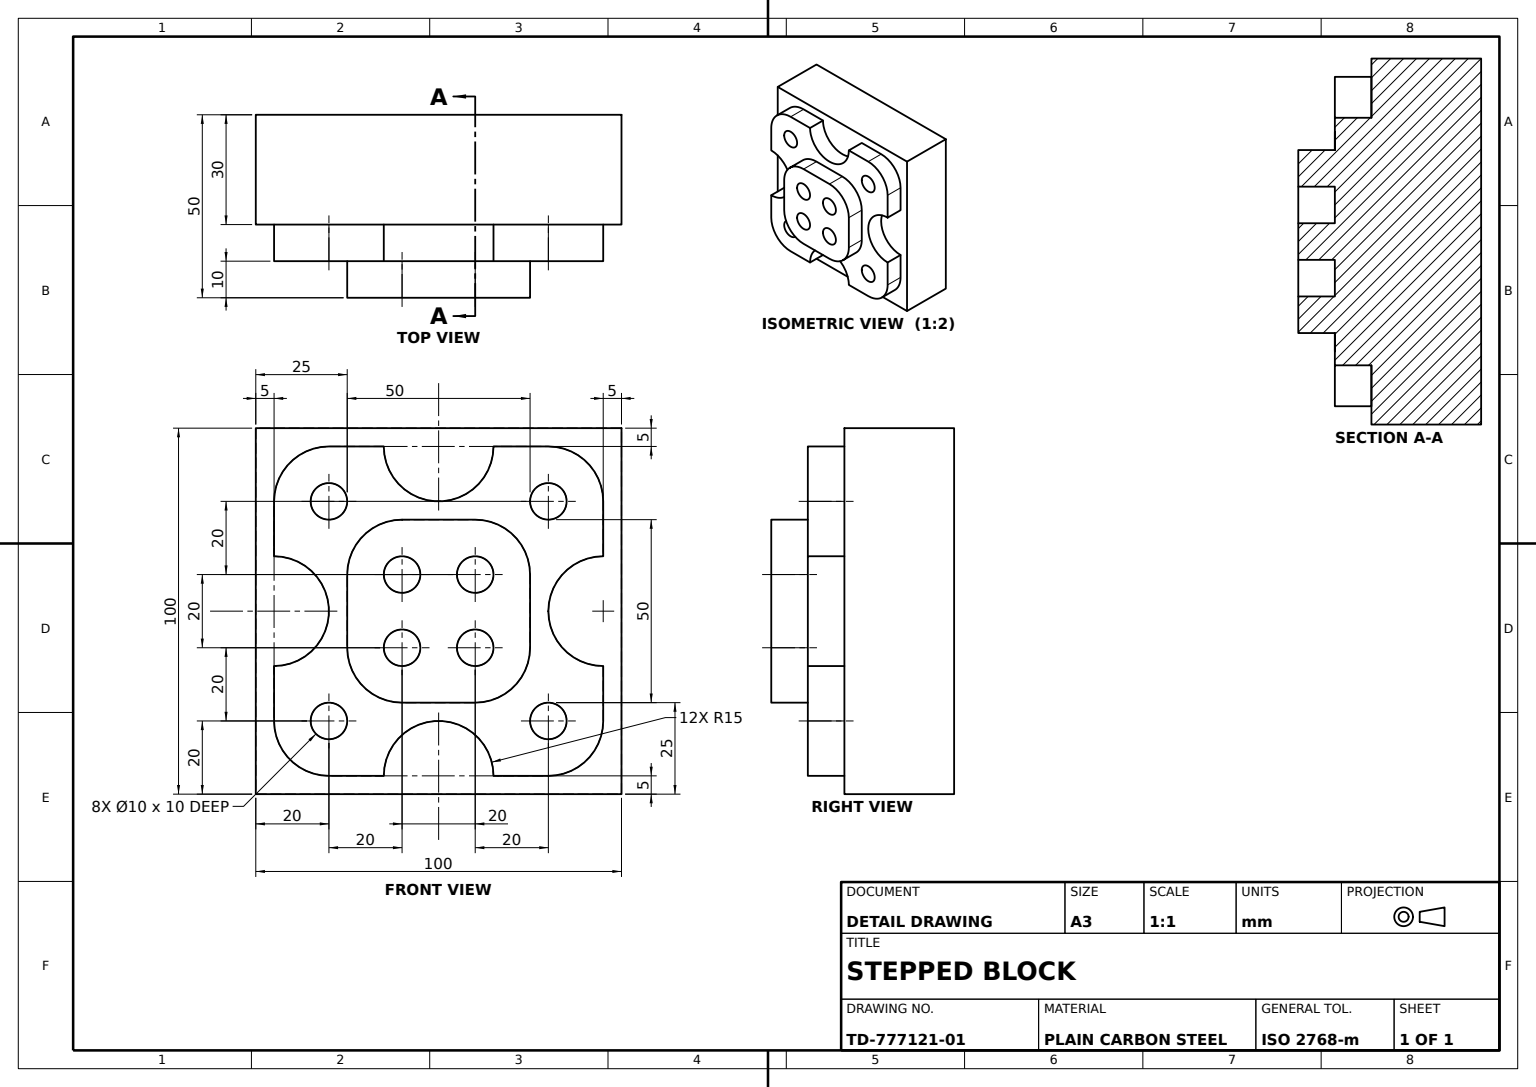
ISO-10303-21;
HEADER;
FILE_DESCRIPTION((''),'2;1');
FILE_NAME('','',(''),(''),'','','');
FILE_SCHEMA(('AUTOMOTIVE_DESIGN'));
ENDSEC;
DATA;
#1=APPLICATION_CONTEXT('');
#2=PRODUCT_CONTEXT('',#1,'mechanical');
#3=PRODUCT('','','',(#2));
#4=PRODUCT_DEFINITION_FORMATION('','',#3);
#5=PRODUCT_DEFINITION_CONTEXT('',#1,'design');
#6=PRODUCT_DEFINITION('','',#4,#5);
#7=PRODUCT_DEFINITION_SHAPE('','',#6);
#8=(LENGTH_UNIT()NAMED_UNIT(*)SI_UNIT(.MILLI.,.METRE.));
#9=(NAMED_UNIT(*)PLANE_ANGLE_UNIT()SI_UNIT($,.RADIAN.));
#10=(NAMED_UNIT(*)SI_UNIT($,.STERADIAN.)SOLID_ANGLE_UNIT());
#11=UNCERTAINTY_MEASURE_WITH_UNIT(LENGTH_MEASURE(1.E-05),#8,'distance_accuracy_value','');
#12=(GEOMETRIC_REPRESENTATION_CONTEXT(3)GLOBAL_UNCERTAINTY_ASSIGNED_CONTEXT((#11))GLOBAL_UNIT_ASSIGNED_CONTEXT((#8,#9,#10))REPRESENTATION_CONTEXT('',''));
#13=CARTESIAN_POINT('',(35.,-5.,30.));
#14=VERTEX_POINT('',#13);
#15=CARTESIAN_POINT('',(20.,-5.,30.));
#16=VERTEX_POINT('',#15);
#17=DIRECTION('',(-1.,0.,0.));
#18=VECTOR('',#17,1000.);
#19=LINE('',#15,#18);
#20=EDGE_CURVE('',#14,#16,#19,.T.);
#21=ORIENTED_EDGE('',*,*,#20,.T.);
#22=CARTESIAN_POINT('',(20.,-5.,40.));
#23=VERTEX_POINT('',#22);
#24=DIRECTION('',(0.,0.,-1.));
#25=VECTOR('',#24,1000.);
#26=LINE('',#22,#25);
#27=EDGE_CURVE('',#23,#16,#26,.T.);
#28=ORIENTED_EDGE('',*,*,#27,.F.);
#29=CARTESIAN_POINT('',(35.,-5.,40.));
#30=VERTEX_POINT('',#29);
#31=LINE('',#22,#18);
#32=EDGE_CURVE('',#30,#23,#31,.T.);
#33=ORIENTED_EDGE('',*,*,#32,.F.);
#34=LINE('',#29,#25);
#35=EDGE_CURVE('',#30,#14,#34,.T.);
#36=ORIENTED_EDGE('',*,*,#35,.T.);
#37=EDGE_LOOP('',(#21,#28,#33,#36));
#38=FACE_OUTER_BOUND('',#37,.T.);
#39=DIRECTION('',(0.,-1.,0.));
#40=AXIS2_PLACEMENT_3D('',#22,#39,#24);
#41=PLANE('',#40);
#42=ADVANCED_FACE('',(#38),#41,.F.);
#43=CARTESIAN_POINT('',(25.,-40.,40.));
#44=VERTEX_POINT('',#43);
#45=CARTESIAN_POINT('',(25.,-60.,40.));
#46=VERTEX_POINT('',#45);
#47=VECTOR('',#39,1000.);
#48=LINE('',#43,#47);
#49=EDGE_CURVE('',#44,#46,#48,.T.);
#50=ORIENTED_EDGE('',*,*,#49,.T.);
#51=CARTESIAN_POINT('',(25.,-60.,50.));
#52=VERTEX_POINT('',#51);
#53=LINE('',#51,#25);
#54=EDGE_CURVE('',#52,#46,#53,.T.);
#55=ORIENTED_EDGE('',*,*,#54,.F.);
#56=CARTESIAN_POINT('',(25.,-40.,50.));
#57=VERTEX_POINT('',#56);
#58=LINE('',#56,#47);
#59=EDGE_CURVE('',#57,#52,#58,.T.);
#60=ORIENTED_EDGE('',*,*,#59,.F.);
#61=LINE('',#56,#25);
#62=EDGE_CURVE('',#57,#44,#61,.T.);
#63=ORIENTED_EDGE('',*,*,#62,.T.);
#64=EDGE_LOOP('',(#50,#55,#60,#63));
#65=FACE_OUTER_BOUND('',#64,.T.);
#66=DIRECTION('',(1.,0.,0.));
#67=DIRECTION('',(0.,1.,0.));
#68=AXIS2_PLACEMENT_3D('',#56,#66,#67);
#69=PLANE('',#68);
#70=ADVANCED_FACE('',(#65),#69,.F.);
#71=CARTESIAN_POINT('',(75.,-20.,30.));
#72=VERTEX_POINT('',#71);
#73=CARTESIAN_POINT('',(75.,-20.,40.));
#74=VERTEX_POINT('',#73);
#75=DIRECTION('',(0.,0.,1.));
#76=VECTOR('',#75,1000.);
#77=LINE('',#71,#76);
#78=EDGE_CURVE('',#72,#74,#77,.T.);
#79=ORIENTED_EDGE('',*,*,#78,.T.);
#80=CARTESIAN_POINT('',(85.,-20.,40.));
#81=VERTEX_POINT('',#80);
#82=CARTESIAN_POINT('',(80.,-20.,40.));
#83=AXIS2_PLACEMENT_3D('',#82,#75,#66);
#84=CIRCLE('',#83,5.);
#85=EDGE_CURVE('',#74,#81,#84,.T.);
#86=ORIENTED_EDGE('',*,*,#85,.T.);
#87=CARTESIAN_POINT('',(85.,-20.,30.));
#88=VERTEX_POINT('',#87);
#89=LINE('',#87,#76);
#90=EDGE_CURVE('',#88,#81,#89,.T.);
#91=ORIENTED_EDGE('',*,*,#90,.F.);
#92=CARTESIAN_POINT('',(80.,-20.,30.));
#93=AXIS2_PLACEMENT_3D('',#92,#75,#66);
#94=CIRCLE('',#93,5.);
#95=EDGE_CURVE('',#72,#88,#94,.T.);
#96=ORIENTED_EDGE('',*,*,#95,.F.);
#97=EDGE_LOOP('',(#79,#86,#91,#96));
#98=FACE_OUTER_BOUND('',#97,.T.);
#99=CYLINDRICAL_SURFACE('',#93,5.);
#100=ADVANCED_FACE('',(#98),#99,.F.);
#101=CARTESIAN_POINT('',(65.,-5.,40.));
#102=VERTEX_POINT('',#101);
#103=CARTESIAN_POINT('',(50.,-5.,40.));
#104=AXIS2_PLACEMENT_3D('',#103,#24,#66);
#105=CIRCLE('',#104,15.);
#106=EDGE_CURVE('',#102,#30,#105,.T.);
#107=ORIENTED_EDGE('',*,*,#106,.F.);
#108=CARTESIAN_POINT('',(65.,-5.,30.));
#109=VERTEX_POINT('',#108);
#110=LINE('',#101,#25);
#111=EDGE_CURVE('',#102,#109,#110,.T.);
#112=ORIENTED_EDGE('',*,*,#111,.T.);
#113=CARTESIAN_POINT('',(50.,-5.,30.));
#114=AXIS2_PLACEMENT_3D('',#113,#24,#66);
#115=CIRCLE('',#114,15.);
#116=EDGE_CURVE('',#109,#14,#115,.T.);
#117=ORIENTED_EDGE('',*,*,#116,.T.);
#118=ORIENTED_EDGE('',*,*,#35,.F.);
#119=EDGE_LOOP('',(#107,#112,#117,#118));
#120=FACE_OUTER_BOUND('',#119,.T.);
#121=AXIS2_PLACEMENT_3D('',#103,#24,#17);
#122=CYLINDRICAL_SURFACE('',#121,15.);
#123=ADVANCED_FACE('',(#120),#122,.F.);
#124=CARTESIAN_POINT('',(65.,-40.,40.));
#125=VERTEX_POINT('',#124);
#126=CARTESIAN_POINT('',(55.,-40.,40.));
#127=VERTEX_POINT('',#126);
#128=CARTESIAN_POINT('',(60.,-40.,40.));
#129=AXIS2_PLACEMENT_3D('',#128,#75,#66);
#130=CIRCLE('',#129,5.);
#131=EDGE_CURVE('',#125,#127,#130,.T.);
#132=ORIENTED_EDGE('',*,*,#131,.T.);
#133=EDGE_CURVE('',#127,#125,#130,.T.);
#134=ORIENTED_EDGE('',*,*,#133,.T.);
#135=EDGE_LOOP('',(#132,#134));
#136=FACE_OUTER_BOUND('',#135,.T.);
#137=PLANE('',#129);
#138=ADVANCED_FACE('',(#136),#137,.T.);
#139=CARTESIAN_POINT('',(80.,-5.,30.));
#140=VERTEX_POINT('',#139);
#141=LINE('',#108,#18);
#142=EDGE_CURVE('',#140,#109,#141,.T.);
#143=ORIENTED_EDGE('',*,*,#142,.T.);
#144=ORIENTED_EDGE('',*,*,#111,.F.);
#145=CARTESIAN_POINT('',(80.,-5.,40.));
#146=VERTEX_POINT('',#145);
#147=LINE('',#101,#18);
#148=EDGE_CURVE('',#146,#102,#147,.T.);
#149=ORIENTED_EDGE('',*,*,#148,.F.);
#150=LINE('',#145,#25);
#151=EDGE_CURVE('',#146,#140,#150,.T.);
#152=ORIENTED_EDGE('',*,*,#151,.T.);
#153=EDGE_LOOP('',(#143,#144,#149,#152));
#154=FACE_OUTER_BOUND('',#153,.T.);
#155=AXIS2_PLACEMENT_3D('',#101,#39,#24);
#156=PLANE('',#155);
#157=ADVANCED_FACE('',(#154),#156,.F.);
#158=CARTESIAN_POINT('',(85.,-80.,40.));
#159=VERTEX_POINT('',#158);
#160=CARTESIAN_POINT('',(75.,-80.,40.));
#161=VERTEX_POINT('',#160);
#162=CARTESIAN_POINT('',(80.,-80.,40.));
#163=AXIS2_PLACEMENT_3D('',#162,#75,#66);
#164=CIRCLE('',#163,5.);
#165=EDGE_CURVE('',#159,#161,#164,.T.);
#166=ORIENTED_EDGE('',*,*,#165,.T.);
#167=CARTESIAN_POINT('',(75.,-80.,30.));
#168=VERTEX_POINT('',#167);
#169=LINE('',#167,#76);
#170=EDGE_CURVE('',#168,#161,#169,.T.);
#171=ORIENTED_EDGE('',*,*,#170,.F.);
#172=CARTESIAN_POINT('',(85.,-80.,30.));
#173=VERTEX_POINT('',#172);
#174=CARTESIAN_POINT('',(80.,-80.,30.));
#175=AXIS2_PLACEMENT_3D('',#174,#75,#66);
#176=CIRCLE('',#175,5.);
#177=EDGE_CURVE('',#173,#168,#176,.T.);
#178=ORIENTED_EDGE('',*,*,#177,.F.);
#179=LINE('',#172,#76);
#180=EDGE_CURVE('',#173,#159,#179,.T.);
#181=ORIENTED_EDGE('',*,*,#180,.T.);
#182=EDGE_LOOP('',(#166,#171,#178,#181));
#183=FACE_OUTER_BOUND('',#182,.T.);
#184=CYLINDRICAL_SURFACE('',#175,5.);
#185=ADVANCED_FACE('',(#183),#184,.F.);
#186=CARTESIAN_POINT('',(40.,-75.,50.));
#187=VERTEX_POINT('',#186);
#188=CARTESIAN_POINT('',(60.,-75.,50.));
#189=VERTEX_POINT('',#188);
#190=VECTOR('',#66,1000.);
#191=LINE('',#186,#190);
#192=EDGE_CURVE('',#187,#189,#191,.T.);
#193=ORIENTED_EDGE('',*,*,#192,.F.);
#194=CARTESIAN_POINT('',(40.,-75.,40.));
#195=VERTEX_POINT('',#194);
#196=LINE('',#186,#25);
#197=EDGE_CURVE('',#187,#195,#196,.T.);
#198=ORIENTED_EDGE('',*,*,#197,.T.);
#199=CARTESIAN_POINT('',(60.,-75.,40.));
#200=VERTEX_POINT('',#199);
#201=LINE('',#194,#190);
#202=EDGE_CURVE('',#195,#200,#201,.T.);
#203=ORIENTED_EDGE('',*,*,#202,.T.);
#204=LINE('',#188,#25);
#205=EDGE_CURVE('',#189,#200,#204,.T.);
#206=ORIENTED_EDGE('',*,*,#205,.F.);
#207=EDGE_LOOP('',(#193,#198,#203,#206));
#208=FACE_OUTER_BOUND('',#207,.T.);
#209=AXIS2_PLACEMENT_3D('',#186,#67,#75);
#210=PLANE('',#209);
#211=ADVANCED_FACE('',(#208),#210,.F.);
#212=CARTESIAN_POINT('',(100.,-100.,30.));
#213=VERTEX_POINT('',#212);
#214=CARTESIAN_POINT('',(100.,0.,30.));
#215=VERTEX_POINT('',#214);
#216=VECTOR('',#67,1000.);
#217=LINE('',#212,#216);
#218=EDGE_CURVE('',#213,#215,#217,.T.);
#219=ORIENTED_EDGE('',*,*,#218,.T.);
#220=CARTESIAN_POINT('',(0.,0.,30.));
#221=VERTEX_POINT('',#220);
#222=LINE('',#214,#18);
#223=EDGE_CURVE('',#215,#221,#222,.T.);
#224=ORIENTED_EDGE('',*,*,#223,.T.);
#225=CARTESIAN_POINT('',(0.,-100.,30.));
#226=VERTEX_POINT('',#225);
#227=LINE('',#220,#47);
#228=EDGE_CURVE('',#221,#226,#227,.T.);
#229=ORIENTED_EDGE('',*,*,#228,.T.);
#230=LINE('',#225,#190);
#231=EDGE_CURVE('',#226,#213,#230,.T.);
#232=ORIENTED_EDGE('',*,*,#231,.T.);
#233=EDGE_LOOP('',(#219,#224,#229,#232));
#234=FACE_OUTER_BOUND('',#233,.T.);
#235=CARTESIAN_POINT('',(5.,-20.,30.));
#236=VERTEX_POINT('',#235);
#237=CARTESIAN_POINT('',(5.,-35.,30.));
#238=VERTEX_POINT('',#237);
#239=LINE('',#235,#47);
#240=EDGE_CURVE('',#236,#238,#239,.T.);
#241=ORIENTED_EDGE('',*,*,#240,.F.);
#242=CARTESIAN_POINT('',(20.,-20.,30.));
#243=AXIS2_PLACEMENT_3D('',#242,#75,#66);
#244=CIRCLE('',#243,15.);
#245=EDGE_CURVE('',#16,#236,#244,.T.);
#246=ORIENTED_EDGE('',*,*,#245,.F.);
#247=ORIENTED_EDGE('',*,*,#20,.F.);
#248=ORIENTED_EDGE('',*,*,#116,.F.);
#249=ORIENTED_EDGE('',*,*,#142,.F.);
#250=CARTESIAN_POINT('',(95.,-20.,30.));
#251=VERTEX_POINT('',#250);
#252=CIRCLE('',#93,15.);
#253=EDGE_CURVE('',#251,#140,#252,.T.);
#254=ORIENTED_EDGE('',*,*,#253,.F.);
#255=CARTESIAN_POINT('',(95.,-35.,30.));
#256=VERTEX_POINT('',#255);
#257=LINE('',#250,#216);
#258=EDGE_CURVE('',#256,#251,#257,.T.);
#259=ORIENTED_EDGE('',*,*,#258,.F.);
#260=CARTESIAN_POINT('',(80.,-50.,30.));
#261=VERTEX_POINT('',#260);
#262=CARTESIAN_POINT('',(95.,-50.,30.));
#263=AXIS2_PLACEMENT_3D('',#262,#24,#66);
#264=CIRCLE('',#263,15.);
#265=EDGE_CURVE('',#261,#256,#264,.T.);
#266=ORIENTED_EDGE('',*,*,#265,.F.);
#267=CARTESIAN_POINT('',(95.,-65.,30.));
#268=VERTEX_POINT('',#267);
#269=EDGE_CURVE('',#268,#261,#264,.T.);
#270=ORIENTED_EDGE('',*,*,#269,.F.);
#271=CARTESIAN_POINT('',(95.,-80.,30.));
#272=VERTEX_POINT('',#271);
#273=LINE('',#267,#216);
#274=EDGE_CURVE('',#272,#268,#273,.T.);
#275=ORIENTED_EDGE('',*,*,#274,.F.);
#276=CARTESIAN_POINT('',(80.,-95.,30.));
#277=VERTEX_POINT('',#276);
#278=CIRCLE('',#175,15.);
#279=EDGE_CURVE('',#277,#272,#278,.T.);
#280=ORIENTED_EDGE('',*,*,#279,.F.);
#281=CARTESIAN_POINT('',(65.,-95.,30.));
#282=VERTEX_POINT('',#281);
#283=LINE('',#281,#190);
#284=EDGE_CURVE('',#282,#277,#283,.T.);
#285=ORIENTED_EDGE('',*,*,#284,.F.);
#286=CARTESIAN_POINT('',(35.,-95.,30.));
#287=VERTEX_POINT('',#286);
#288=CARTESIAN_POINT('',(50.,-95.,30.));
#289=AXIS2_PLACEMENT_3D('',#288,#24,#66);
#290=CIRCLE('',#289,15.);
#291=EDGE_CURVE('',#287,#282,#290,.T.);
#292=ORIENTED_EDGE('',*,*,#291,.F.);
#293=CARTESIAN_POINT('',(20.,-95.,30.));
#294=VERTEX_POINT('',#293);
#295=LINE('',#293,#190);
#296=EDGE_CURVE('',#294,#287,#295,.T.);
#297=ORIENTED_EDGE('',*,*,#296,.F.);
#298=CARTESIAN_POINT('',(5.,-80.,30.));
#299=VERTEX_POINT('',#298);
#300=CARTESIAN_POINT('',(20.,-80.,30.));
#301=AXIS2_PLACEMENT_3D('',#300,#75,#17);
#302=CIRCLE('',#301,15.);
#303=EDGE_CURVE('',#299,#294,#302,.T.);
#304=ORIENTED_EDGE('',*,*,#303,.F.);
#305=CARTESIAN_POINT('',(5.,-65.,30.));
#306=VERTEX_POINT('',#305);
#307=LINE('',#305,#47);
#308=EDGE_CURVE('',#306,#299,#307,.T.);
#309=ORIENTED_EDGE('',*,*,#308,.F.);
#310=CARTESIAN_POINT('',(5.,-50.,30.));
#311=AXIS2_PLACEMENT_3D('',#310,#24,#66);
#312=CIRCLE('',#311,15.);
#313=EDGE_CURVE('',#238,#306,#312,.T.);
#314=ORIENTED_EDGE('',*,*,#313,.F.);
#315=EDGE_LOOP('',(#241,#246,#247,#248,#249,#254,#259,#266,#270,#275,#280,#285,#292,#297,#304,#309,#314));
#316=FACE_BOUND('',#315,.T.);
#317=AXIS2_PLACEMENT_3D('',#220,#75,#66);
#318=PLANE('',#317);
#319=ADVANCED_FACE('',(#234,#316),#318,.T.);
#320=CARTESIAN_POINT('',(95.,-20.,40.));
#321=VERTEX_POINT('',#320);
#322=LINE('',#320,#25);
#323=EDGE_CURVE('',#321,#251,#322,.T.);
#324=ORIENTED_EDGE('',*,*,#323,.F.);
#325=CARTESIAN_POINT('',(95.,-35.,40.));
#326=VERTEX_POINT('',#325);
#327=LINE('',#320,#216);
#328=EDGE_CURVE('',#326,#321,#327,.T.);
#329=ORIENTED_EDGE('',*,*,#328,.F.);
#330=LINE('',#325,#25);
#331=EDGE_CURVE('',#326,#256,#330,.T.);
#332=ORIENTED_EDGE('',*,*,#331,.T.);
#333=ORIENTED_EDGE('',*,*,#258,.T.);
#334=EDGE_LOOP('',(#324,#329,#332,#333));
#335=FACE_OUTER_BOUND('',#334,.T.);
#336=AXIS2_PLACEMENT_3D('',#320,#17,#75);
#337=PLANE('',#336);
#338=ADVANCED_FACE('',(#335),#337,.F.);
#339=ORIENTED_EDGE('',*,*,#313,.T.);
#340=CARTESIAN_POINT('',(5.,-65.,40.));
#341=VERTEX_POINT('',#340);
#342=LINE('',#340,#25);
#343=EDGE_CURVE('',#341,#306,#342,.T.);
#344=ORIENTED_EDGE('',*,*,#343,.F.);
#345=CARTESIAN_POINT('',(5.,-35.,40.));
#346=VERTEX_POINT('',#345);
#347=CARTESIAN_POINT('',(5.,-50.,40.));
#348=AXIS2_PLACEMENT_3D('',#347,#24,#66);
#349=CIRCLE('',#348,15.);
#350=EDGE_CURVE('',#346,#341,#349,.T.);
#351=ORIENTED_EDGE('',*,*,#350,.F.);
#352=LINE('',#345,#25);
#353=EDGE_CURVE('',#346,#238,#352,.T.);
#354=ORIENTED_EDGE('',*,*,#353,.T.);
#355=EDGE_LOOP('',(#339,#344,#351,#354));
#356=FACE_OUTER_BOUND('',#355,.T.);
#357=AXIS2_PLACEMENT_3D('',#347,#24,#17);
#358=CYLINDRICAL_SURFACE('',#357,15.);
#359=ADVANCED_FACE('',(#356),#358,.F.);
#360=CARTESIAN_POINT('',(5.,-80.,40.));
#361=VERTEX_POINT('',#360);
#362=LINE('',#360,#25);
#363=EDGE_CURVE('',#361,#299,#362,.T.);
#364=ORIENTED_EDGE('',*,*,#363,.F.);
#365=LINE('',#340,#47);
#366=EDGE_CURVE('',#341,#361,#365,.T.);
#367=ORIENTED_EDGE('',*,*,#366,.F.);
#368=ORIENTED_EDGE('',*,*,#343,.T.);
#369=ORIENTED_EDGE('',*,*,#308,.T.);
#370=EDGE_LOOP('',(#364,#367,#368,#369));
#371=FACE_OUTER_BOUND('',#370,.T.);
#372=AXIS2_PLACEMENT_3D('',#340,#66,#67);
#373=PLANE('',#372);
#374=ADVANCED_FACE('',(#371),#373,.F.);
#375=CARTESIAN_POINT('',(80.,-50.,40.));
#376=VERTEX_POINT('',#375);
#377=LINE('',#375,#25);
#378=EDGE_CURVE('',#376,#261,#377,.T.);
#379=ORIENTED_EDGE('',*,*,#378,.T.);
#380=ORIENTED_EDGE('',*,*,#265,.T.);
#381=ORIENTED_EDGE('',*,*,#331,.F.);
#382=CARTESIAN_POINT('',(95.,-50.,40.));
#383=AXIS2_PLACEMENT_3D('',#382,#24,#66);
#384=CIRCLE('',#383,15.);
#385=EDGE_CURVE('',#376,#326,#384,.T.);
#386=ORIENTED_EDGE('',*,*,#385,.F.);
#387=EDGE_LOOP('',(#379,#380,#381,#386));
#388=FACE_OUTER_BOUND('',#387,.T.);
#389=AXIS2_PLACEMENT_3D('',#382,#24,#17);
#390=CYLINDRICAL_SURFACE('',#389,15.);
#391=ADVANCED_FACE('',(#388),#390,.F.);
#392=CARTESIAN_POINT('',(60.,-25.,50.));
#393=VERTEX_POINT('',#392);
#394=CARTESIAN_POINT('',(60.,-25.,40.));
#395=VERTEX_POINT('',#394);
#396=LINE('',#392,#25);
#397=EDGE_CURVE('',#393,#395,#396,.T.);
#398=ORIENTED_EDGE('',*,*,#397,.T.);
#399=CARTESIAN_POINT('',(40.,-25.,40.));
#400=VERTEX_POINT('',#399);
#401=LINE('',#399,#18);
#402=EDGE_CURVE('',#395,#400,#401,.T.);
#403=ORIENTED_EDGE('',*,*,#402,.T.);
#404=CARTESIAN_POINT('',(40.,-25.,50.));
#405=VERTEX_POINT('',#404);
#406=LINE('',#404,#25);
#407=EDGE_CURVE('',#405,#400,#406,.T.);
#408=ORIENTED_EDGE('',*,*,#407,.F.);
#409=LINE('',#404,#18);
#410=EDGE_CURVE('',#393,#405,#409,.T.);
#411=ORIENTED_EDGE('',*,*,#410,.F.);
#412=EDGE_LOOP('',(#398,#403,#408,#411));
#413=FACE_OUTER_BOUND('',#412,.T.);
#414=AXIS2_PLACEMENT_3D('',#404,#39,#24);
#415=PLANE('',#414);
#416=ADVANCED_FACE('',(#413),#415,.F.);
#417=ORIENTED_EDGE('',*,*,#165,.F.);
#418=EDGE_CURVE('',#161,#159,#164,.T.);
#419=ORIENTED_EDGE('',*,*,#418,.F.);
#420=EDGE_LOOP('',(#417,#419));
#421=FACE_BOUND('',#420,.T.);
#422=CARTESIAN_POINT('',(25.,-80.,40.));
#423=VERTEX_POINT('',#422);
#424=CARTESIAN_POINT('',(15.,-80.,40.));
#425=VERTEX_POINT('',#424);
#426=CARTESIAN_POINT('',(20.,-80.,40.));
#427=AXIS2_PLACEMENT_3D('',#426,#75,#66);
#428=CIRCLE('',#427,5.);
#429=EDGE_CURVE('',#423,#425,#428,.T.);
#430=ORIENTED_EDGE('',*,*,#429,.F.);
#431=EDGE_CURVE('',#425,#423,#428,.T.);
#432=ORIENTED_EDGE('',*,*,#431,.F.);
#433=EDGE_LOOP('',(#430,#432));
#434=FACE_BOUND('',#433,.T.);
#435=ORIENTED_EDGE('',*,*,#350,.T.);
#436=ORIENTED_EDGE('',*,*,#366,.T.);
#437=CARTESIAN_POINT('',(20.,-95.,40.));
#438=VERTEX_POINT('',#437);
#439=AXIS2_PLACEMENT_3D('',#426,#75,#17);
#440=CIRCLE('',#439,15.);
#441=EDGE_CURVE('',#361,#438,#440,.T.);
#442=ORIENTED_EDGE('',*,*,#441,.T.);
#443=CARTESIAN_POINT('',(35.,-95.,40.));
#444=VERTEX_POINT('',#443);
#445=LINE('',#437,#190);
#446=EDGE_CURVE('',#438,#444,#445,.T.);
#447=ORIENTED_EDGE('',*,*,#446,.T.);
#448=CARTESIAN_POINT('',(65.,-95.,40.));
#449=VERTEX_POINT('',#448);
#450=CARTESIAN_POINT('',(50.,-95.,40.));
#451=AXIS2_PLACEMENT_3D('',#450,#24,#66);
#452=CIRCLE('',#451,15.);
#453=EDGE_CURVE('',#444,#449,#452,.T.);
#454=ORIENTED_EDGE('',*,*,#453,.T.);
#455=CARTESIAN_POINT('',(80.,-95.,40.));
#456=VERTEX_POINT('',#455);
#457=LINE('',#448,#190);
#458=EDGE_CURVE('',#449,#456,#457,.T.);
#459=ORIENTED_EDGE('',*,*,#458,.T.);
#460=CARTESIAN_POINT('',(95.,-80.,40.));
#461=VERTEX_POINT('',#460);
#462=CIRCLE('',#163,15.);
#463=EDGE_CURVE('',#456,#461,#462,.T.);
#464=ORIENTED_EDGE('',*,*,#463,.T.);
#465=CARTESIAN_POINT('',(95.,-65.,40.));
#466=VERTEX_POINT('',#465);
#467=LINE('',#465,#216);
#468=EDGE_CURVE('',#461,#466,#467,.T.);
#469=ORIENTED_EDGE('',*,*,#468,.T.);
#470=EDGE_CURVE('',#466,#376,#384,.T.);
#471=ORIENTED_EDGE('',*,*,#470,.T.);
#472=ORIENTED_EDGE('',*,*,#385,.T.);
#473=ORIENTED_EDGE('',*,*,#328,.T.);
#474=CIRCLE('',#83,15.);
#475=EDGE_CURVE('',#321,#146,#474,.T.);
#476=ORIENTED_EDGE('',*,*,#475,.T.);
#477=ORIENTED_EDGE('',*,*,#148,.T.);
#478=ORIENTED_EDGE('',*,*,#106,.T.);
#479=ORIENTED_EDGE('',*,*,#32,.T.);
#480=CARTESIAN_POINT('',(5.,-20.,40.));
#481=VERTEX_POINT('',#480);
#482=CARTESIAN_POINT('',(20.,-20.,40.));
#483=AXIS2_PLACEMENT_3D('',#482,#75,#66);
#484=CIRCLE('',#483,15.);
#485=EDGE_CURVE('',#23,#481,#484,.T.);
#486=ORIENTED_EDGE('',*,*,#485,.T.);
#487=LINE('',#480,#47);
#488=EDGE_CURVE('',#481,#346,#487,.T.);
#489=ORIENTED_EDGE('',*,*,#488,.T.);
#490=EDGE_LOOP('',(#435,#436,#442,#447,#454,#459,#464,#469,#471,#472,#473,#476,#477,#478,#479,#486,#489));
#491=FACE_OUTER_BOUND('',#490,.T.);
#492=CARTESIAN_POINT('',(15.,-20.,40.));
#493=VERTEX_POINT('',#492);
#494=CARTESIAN_POINT('',(25.,-20.,40.));
#495=VERTEX_POINT('',#494);
#496=CIRCLE('',#483,5.);
#497=EDGE_CURVE('',#493,#495,#496,.T.);
#498=ORIENTED_EDGE('',*,*,#497,.F.);
#499=EDGE_CURVE('',#495,#493,#496,.T.);
#500=ORIENTED_EDGE('',*,*,#499,.F.);
#501=EDGE_LOOP('',(#498,#500));
#502=FACE_BOUND('',#501,.T.);
#503=CARTESIAN_POINT('',(40.,-40.,40.));
#504=AXIS2_PLACEMENT_3D('',#503,#75,#66);
#505=CIRCLE('',#504,15.);
#506=EDGE_CURVE('',#400,#44,#505,.T.);
#507=ORIENTED_EDGE('',*,*,#506,.F.);
#508=ORIENTED_EDGE('',*,*,#402,.F.);
#509=CARTESIAN_POINT('',(75.,-40.,40.));
#510=VERTEX_POINT('',#509);
#511=CIRCLE('',#129,15.);
#512=EDGE_CURVE('',#510,#395,#511,.T.);
#513=ORIENTED_EDGE('',*,*,#512,.F.);
#514=CARTESIAN_POINT('',(75.,-60.,40.));
#515=VERTEX_POINT('',#514);
#516=LINE('',#509,#216);
#517=EDGE_CURVE('',#515,#510,#516,.T.);
#518=ORIENTED_EDGE('',*,*,#517,.F.);
#519=CARTESIAN_POINT('',(60.,-60.,40.));
#520=AXIS2_PLACEMENT_3D('',#519,#75,#66);
#521=CIRCLE('',#520,15.);
#522=EDGE_CURVE('',#200,#515,#521,.T.);
#523=ORIENTED_EDGE('',*,*,#522,.F.);
#524=ORIENTED_EDGE('',*,*,#202,.F.);
#525=CARTESIAN_POINT('',(40.,-60.,40.));
#526=AXIS2_PLACEMENT_3D('',#525,#75,#66);
#527=CIRCLE('',#526,15.);
#528=EDGE_CURVE('',#46,#195,#527,.T.);
#529=ORIENTED_EDGE('',*,*,#528,.F.);
#530=ORIENTED_EDGE('',*,*,#49,.F.);
#531=EDGE_LOOP('',(#507,#508,#513,#518,#523,#524,#529,#530));
#532=FACE_BOUND('',#531,.T.);
#533=ORIENTED_EDGE('',*,*,#85,.F.);
#534=EDGE_CURVE('',#81,#74,#84,.T.);
#535=ORIENTED_EDGE('',*,*,#534,.F.);
#536=EDGE_LOOP('',(#533,#535));
#537=FACE_BOUND('',#536,.T.);
#538=AXIS2_PLACEMENT_3D('',#426,#24,#17);
#539=PLANE('',#538);
#540=ADVANCED_FACE('',(#421,#434,#491,#502,#532,#537),#539,.F.);
#541=CARTESIAN_POINT('',(35.,-60.,40.));
#542=VERTEX_POINT('',#541);
#543=CARTESIAN_POINT('',(35.,-60.,50.));
#544=VERTEX_POINT('',#543);
#545=LINE('',#541,#76);
#546=EDGE_CURVE('',#542,#544,#545,.T.);
#547=ORIENTED_EDGE('',*,*,#546,.F.);
#548=CARTESIAN_POINT('',(45.,-60.,40.));
#549=VERTEX_POINT('',#548);
#550=CIRCLE('',#526,5.);
#551=EDGE_CURVE('',#549,#542,#550,.T.);
#552=ORIENTED_EDGE('',*,*,#551,.F.);
#553=CARTESIAN_POINT('',(45.,-60.,50.));
#554=VERTEX_POINT('',#553);
#555=LINE('',#548,#76);
#556=EDGE_CURVE('',#549,#554,#555,.T.);
#557=ORIENTED_EDGE('',*,*,#556,.T.);
#558=CARTESIAN_POINT('',(40.,-60.,50.));
#559=AXIS2_PLACEMENT_3D('',#558,#75,#66);
#560=CIRCLE('',#559,5.);
#561=EDGE_CURVE('',#554,#544,#560,.T.);
#562=ORIENTED_EDGE('',*,*,#561,.T.);
#563=EDGE_LOOP('',(#547,#552,#557,#562));
#564=FACE_OUTER_BOUND('',#563,.T.);
#565=CYLINDRICAL_SURFACE('',#526,5.);
#566=ADVANCED_FACE('',(#564),#565,.F.);
#567=ORIENTED_EDGE('',*,*,#458,.F.);
#568=LINE('',#448,#25);
#569=EDGE_CURVE('',#449,#282,#568,.T.);
#570=ORIENTED_EDGE('',*,*,#569,.T.);
#571=ORIENTED_EDGE('',*,*,#284,.T.);
#572=LINE('',#455,#25);
#573=EDGE_CURVE('',#456,#277,#572,.T.);
#574=ORIENTED_EDGE('',*,*,#573,.F.);
#575=EDGE_LOOP('',(#567,#570,#571,#574));
#576=FACE_OUTER_BOUND('',#575,.T.);
#577=AXIS2_PLACEMENT_3D('',#448,#67,#75);
#578=PLANE('',#577);
#579=ADVANCED_FACE('',(#576),#578,.F.);
#580=ORIENTED_EDGE('',*,*,#177,.T.);
#581=EDGE_CURVE('',#168,#173,#176,.T.);
#582=ORIENTED_EDGE('',*,*,#581,.T.);
#583=EDGE_LOOP('',(#580,#582));
#584=FACE_OUTER_BOUND('',#583,.T.);
#585=PLANE('',#175);
#586=ADVANCED_FACE('',(#584),#585,.T.);
#587=ORIENTED_EDGE('',*,*,#78,.F.);
#588=EDGE_CURVE('',#88,#72,#94,.T.);
#589=ORIENTED_EDGE('',*,*,#588,.F.);
#590=ORIENTED_EDGE('',*,*,#90,.T.);
#591=ORIENTED_EDGE('',*,*,#534,.T.);
#592=EDGE_LOOP('',(#587,#589,#590,#591));
#593=FACE_OUTER_BOUND('',#592,.T.);
#594=ADVANCED_FACE('',(#593),#99,.F.);
#595=CARTESIAN_POINT('',(45.,-40.,50.));
#596=VERTEX_POINT('',#595);
#597=CARTESIAN_POINT('',(35.,-40.,50.));
#598=VERTEX_POINT('',#597);
#599=CARTESIAN_POINT('',(40.,-40.,50.));
#600=AXIS2_PLACEMENT_3D('',#599,#75,#66);
#601=CIRCLE('',#600,5.);
#602=EDGE_CURVE('',#596,#598,#601,.T.);
#603=ORIENTED_EDGE('',*,*,#602,.F.);
#604=EDGE_CURVE('',#598,#596,#601,.T.);
#605=ORIENTED_EDGE('',*,*,#604,.F.);
#606=EDGE_LOOP('',(#603,#605));
#607=FACE_BOUND('',#606,.T.);
#608=CARTESIAN_POINT('',(75.,-60.,50.));
#609=VERTEX_POINT('',#608);
#610=CARTESIAN_POINT('',(75.,-40.,50.));
#611=VERTEX_POINT('',#610);
#612=LINE('',#610,#216);
#613=EDGE_CURVE('',#609,#611,#612,.T.);
#614=ORIENTED_EDGE('',*,*,#613,.T.);
#615=CARTESIAN_POINT('',(60.,-40.,50.));
#616=AXIS2_PLACEMENT_3D('',#615,#75,#66);
#617=CIRCLE('',#616,15.);
#618=EDGE_CURVE('',#611,#393,#617,.T.);
#619=ORIENTED_EDGE('',*,*,#618,.T.);
#620=ORIENTED_EDGE('',*,*,#410,.T.);
#621=CIRCLE('',#600,15.);
#622=EDGE_CURVE('',#405,#57,#621,.T.);
#623=ORIENTED_EDGE('',*,*,#622,.T.);
#624=ORIENTED_EDGE('',*,*,#59,.T.);
#625=CIRCLE('',#559,15.);
#626=EDGE_CURVE('',#52,#187,#625,.T.);
#627=ORIENTED_EDGE('',*,*,#626,.T.);
#628=ORIENTED_EDGE('',*,*,#192,.T.);
#629=CARTESIAN_POINT('',(60.,-60.,50.));
#630=AXIS2_PLACEMENT_3D('',#629,#75,#66);
#631=CIRCLE('',#630,15.);
#632=EDGE_CURVE('',#189,#609,#631,.T.);
#633=ORIENTED_EDGE('',*,*,#632,.T.);
#634=EDGE_LOOP('',(#614,#619,#620,#623,#624,#627,#628,#633));
#635=FACE_OUTER_BOUND('',#634,.T.);
#636=CARTESIAN_POINT('',(55.,-40.,50.));
#637=VERTEX_POINT('',#636);
#638=CARTESIAN_POINT('',(65.,-40.,50.));
#639=VERTEX_POINT('',#638);
#640=CIRCLE('',#616,5.);
#641=EDGE_CURVE('',#637,#639,#640,.T.);
#642=ORIENTED_EDGE('',*,*,#641,.F.);
#643=EDGE_CURVE('',#639,#637,#640,.T.);
#644=ORIENTED_EDGE('',*,*,#643,.F.);
#645=EDGE_LOOP('',(#642,#644));
#646=FACE_BOUND('',#645,.T.);
#647=CARTESIAN_POINT('',(65.,-60.,50.));
#648=VERTEX_POINT('',#647);
#649=CARTESIAN_POINT('',(55.,-60.,50.));
#650=VERTEX_POINT('',#649);
#651=CIRCLE('',#630,5.);
#652=EDGE_CURVE('',#648,#650,#651,.T.);
#653=ORIENTED_EDGE('',*,*,#652,.F.);
#654=EDGE_CURVE('',#650,#648,#651,.T.);
#655=ORIENTED_EDGE('',*,*,#654,.F.);
#656=EDGE_LOOP('',(#653,#655));
#657=FACE_BOUND('',#656,.T.);
#658=ORIENTED_EDGE('',*,*,#561,.F.);
#659=EDGE_CURVE('',#544,#554,#560,.T.);
#660=ORIENTED_EDGE('',*,*,#659,.F.);
#661=EDGE_LOOP('',(#658,#660));
#662=FACE_BOUND('',#661,.T.);
#663=PLANE('',#600);
#664=ADVANCED_FACE('',(#607,#635,#646,#657,#662),#663,.T.);
#665=ORIENTED_EDGE('',*,*,#231,.F.);
#666=CARTESIAN_POINT('',(0.,-100.,0.));
#667=VERTEX_POINT('',#666);
#668=LINE('',#225,#25);
#669=EDGE_CURVE('',#226,#667,#668,.T.);
#670=ORIENTED_EDGE('',*,*,#669,.T.);
#671=CARTESIAN_POINT('',(100.,-100.,0.));
#672=VERTEX_POINT('',#671);
#673=LINE('',#666,#190);
#674=EDGE_CURVE('',#667,#672,#673,.T.);
#675=ORIENTED_EDGE('',*,*,#674,.T.);
#676=LINE('',#212,#25);
#677=EDGE_CURVE('',#213,#672,#676,.T.);
#678=ORIENTED_EDGE('',*,*,#677,.F.);
#679=EDGE_LOOP('',(#665,#670,#675,#678));
#680=FACE_OUTER_BOUND('',#679,.T.);
#681=AXIS2_PLACEMENT_3D('',#225,#67,#75);
#682=PLANE('',#681);
#683=ADVANCED_FACE('',(#680),#682,.F.);
#684=ORIENTED_EDGE('',*,*,#551,.T.);
#685=EDGE_CURVE('',#542,#549,#550,.T.);
#686=ORIENTED_EDGE('',*,*,#685,.T.);
#687=EDGE_LOOP('',(#684,#686));
#688=FACE_OUTER_BOUND('',#687,.T.);
#689=PLANE('',#526);
#690=ADVANCED_FACE('',(#688),#689,.T.);
#691=ORIENTED_EDGE('',*,*,#407,.T.);
#692=ORIENTED_EDGE('',*,*,#506,.T.);
#693=ORIENTED_EDGE('',*,*,#62,.F.);
#694=ORIENTED_EDGE('',*,*,#622,.F.);
#695=EDGE_LOOP('',(#691,#692,#693,#694));
#696=FACE_OUTER_BOUND('',#695,.T.);
#697=AXIS2_PLACEMENT_3D('',#599,#24,#17);
#698=CYLINDRICAL_SURFACE('',#697,15.);
#699=ADVANCED_FACE('',(#696),#698,.T.);
#700=ORIENTED_EDGE('',*,*,#517,.T.);
#701=LINE('',#610,#25);
#702=EDGE_CURVE('',#611,#510,#701,.T.);
#703=ORIENTED_EDGE('',*,*,#702,.F.);
#704=ORIENTED_EDGE('',*,*,#613,.F.);
#705=LINE('',#608,#25);
#706=EDGE_CURVE('',#609,#515,#705,.T.);
#707=ORIENTED_EDGE('',*,*,#706,.T.);
#708=EDGE_LOOP('',(#700,#703,#704,#707));
#709=FACE_OUTER_BOUND('',#708,.T.);
#710=AXIS2_PLACEMENT_3D('',#610,#17,#75);
#711=PLANE('',#710);
#712=ADVANCED_FACE('',(#709),#711,.F.);
#713=CARTESIAN_POINT('',(45.,-40.,40.));
#714=VERTEX_POINT('',#713);
#715=LINE('',#713,#76);
#716=EDGE_CURVE('',#714,#596,#715,.T.);
#717=ORIENTED_EDGE('',*,*,#716,.F.);
#718=CARTESIAN_POINT('',(35.,-40.,40.));
#719=VERTEX_POINT('',#718);
#720=CIRCLE('',#504,5.);
#721=EDGE_CURVE('',#719,#714,#720,.T.);
#722=ORIENTED_EDGE('',*,*,#721,.F.);
#723=LINE('',#718,#76);
#724=EDGE_CURVE('',#719,#598,#723,.T.);
#725=ORIENTED_EDGE('',*,*,#724,.T.);
#726=ORIENTED_EDGE('',*,*,#604,.T.);
#727=EDGE_LOOP('',(#717,#722,#725,#726));
#728=FACE_OUTER_BOUND('',#727,.T.);
#729=CYLINDRICAL_SURFACE('',#504,5.);
#730=ADVANCED_FACE('',(#728),#729,.F.);
#731=ORIENTED_EDGE('',*,*,#632,.F.);
#732=ORIENTED_EDGE('',*,*,#205,.T.);
#733=ORIENTED_EDGE('',*,*,#522,.T.);
#734=ORIENTED_EDGE('',*,*,#706,.F.);
#735=EDGE_LOOP('',(#731,#732,#733,#734));
#736=FACE_OUTER_BOUND('',#735,.T.);
#737=AXIS2_PLACEMENT_3D('',#629,#24,#17);
#738=CYLINDRICAL_SURFACE('',#737,15.);
#739=ADVANCED_FACE('',(#736),#738,.T.);
#740=CARTESIAN_POINT('',(65.,-60.,40.));
#741=VERTEX_POINT('',#740);
#742=LINE('',#740,#76);
#743=EDGE_CURVE('',#741,#648,#742,.T.);
#744=ORIENTED_EDGE('',*,*,#743,.F.);
#745=CARTESIAN_POINT('',(55.,-60.,40.));
#746=VERTEX_POINT('',#745);
#747=CIRCLE('',#520,5.);
#748=EDGE_CURVE('',#746,#741,#747,.T.);
#749=ORIENTED_EDGE('',*,*,#748,.F.);
#750=LINE('',#745,#76);
#751=EDGE_CURVE('',#746,#650,#750,.T.);
#752=ORIENTED_EDGE('',*,*,#751,.T.);
#753=ORIENTED_EDGE('',*,*,#654,.T.);
#754=EDGE_LOOP('',(#744,#749,#752,#753));
#755=FACE_OUTER_BOUND('',#754,.T.);
#756=CYLINDRICAL_SURFACE('',#520,5.);
#757=ADVANCED_FACE('',(#755),#756,.F.);
#758=LINE('',#126,#76);
#759=EDGE_CURVE('',#127,#637,#758,.T.);
#760=ORIENTED_EDGE('',*,*,#759,.T.);
#761=ORIENTED_EDGE('',*,*,#641,.T.);
#762=LINE('',#124,#76);
#763=EDGE_CURVE('',#125,#639,#762,.T.);
#764=ORIENTED_EDGE('',*,*,#763,.F.);
#765=ORIENTED_EDGE('',*,*,#133,.F.);
#766=EDGE_LOOP('',(#760,#761,#764,#765));
#767=FACE_OUTER_BOUND('',#766,.T.);
#768=CYLINDRICAL_SURFACE('',#129,5.);
#769=ADVANCED_FACE('',(#767),#768,.F.);
#770=ORIENTED_EDGE('',*,*,#95,.T.);
#771=ORIENTED_EDGE('',*,*,#588,.T.);
#772=EDGE_LOOP('',(#770,#771));
#773=FACE_OUTER_BOUND('',#772,.T.);
#774=PLANE('',#93);
#775=ADVANCED_FACE('',(#773),#774,.T.);
#776=LINE('',#460,#25);
#777=EDGE_CURVE('',#461,#272,#776,.T.);
#778=ORIENTED_EDGE('',*,*,#777,.F.);
#779=ORIENTED_EDGE('',*,*,#463,.F.);
#780=ORIENTED_EDGE('',*,*,#573,.T.);
#781=ORIENTED_EDGE('',*,*,#279,.T.);
#782=EDGE_LOOP('',(#778,#779,#780,#781));
#783=FACE_OUTER_BOUND('',#782,.T.);
#784=AXIS2_PLACEMENT_3D('',#162,#24,#17);
#785=CYLINDRICAL_SURFACE('',#784,15.);
#786=ADVANCED_FACE('',(#783),#785,.T.);
#787=ORIENTED_EDGE('',*,*,#475,.F.);
#788=ORIENTED_EDGE('',*,*,#323,.T.);
#789=ORIENTED_EDGE('',*,*,#253,.T.);
#790=ORIENTED_EDGE('',*,*,#151,.F.);
#791=EDGE_LOOP('',(#787,#788,#789,#790));
#792=FACE_OUTER_BOUND('',#791,.T.);
#793=AXIS2_PLACEMENT_3D('',#82,#24,#17);
#794=CYLINDRICAL_SURFACE('',#793,15.);
#795=ADVANCED_FACE('',(#792),#794,.T.);
#796=LINE('',#437,#25);
#797=EDGE_CURVE('',#438,#294,#796,.T.);
#798=ORIENTED_EDGE('',*,*,#797,.T.);
#799=ORIENTED_EDGE('',*,*,#296,.T.);
#800=LINE('',#443,#25);
#801=EDGE_CURVE('',#444,#287,#800,.T.);
#802=ORIENTED_EDGE('',*,*,#801,.F.);
#803=ORIENTED_EDGE('',*,*,#446,.F.);
#804=EDGE_LOOP('',(#798,#799,#802,#803));
#805=FACE_OUTER_BOUND('',#804,.T.);
#806=AXIS2_PLACEMENT_3D('',#437,#67,#75);
#807=PLANE('',#806);
#808=ADVANCED_FACE('',(#805),#807,.F.);
#809=ORIENTED_EDGE('',*,*,#223,.F.);
#810=CARTESIAN_POINT('',(100.,0.,0.));
#811=VERTEX_POINT('',#810);
#812=LINE('',#214,#25);
#813=EDGE_CURVE('',#215,#811,#812,.T.);
#814=ORIENTED_EDGE('',*,*,#813,.T.);
#815=CARTESIAN_POINT('',(0.,0.,0.));
#816=VERTEX_POINT('',#815);
#817=LINE('',#810,#18);
#818=EDGE_CURVE('',#811,#816,#817,.T.);
#819=ORIENTED_EDGE('',*,*,#818,.T.);
#820=LINE('',#220,#25);
#821=EDGE_CURVE('',#221,#816,#820,.T.);
#822=ORIENTED_EDGE('',*,*,#821,.F.);
#823=EDGE_LOOP('',(#809,#814,#819,#822));
#824=FACE_OUTER_BOUND('',#823,.T.);
#825=AXIS2_PLACEMENT_3D('',#214,#39,#24);
#826=PLANE('',#825);
#827=ADVANCED_FACE('',(#824),#826,.F.);
#828=ORIENTED_EDGE('',*,*,#497,.T.);
#829=CARTESIAN_POINT('',(25.,-20.,30.));
#830=VERTEX_POINT('',#829);
#831=LINE('',#829,#76);
#832=EDGE_CURVE('',#830,#495,#831,.T.);
#833=ORIENTED_EDGE('',*,*,#832,.F.);
#834=CARTESIAN_POINT('',(15.,-20.,30.));
#835=VERTEX_POINT('',#834);
#836=CIRCLE('',#243,5.);
#837=EDGE_CURVE('',#835,#830,#836,.T.);
#838=ORIENTED_EDGE('',*,*,#837,.F.);
#839=LINE('',#834,#76);
#840=EDGE_CURVE('',#835,#493,#839,.T.);
#841=ORIENTED_EDGE('',*,*,#840,.T.);
#842=EDGE_LOOP('',(#828,#833,#838,#841));
#843=FACE_OUTER_BOUND('',#842,.T.);
#844=CYLINDRICAL_SURFACE('',#243,5.);
#845=ADVANCED_FACE('',(#843),#844,.F.);
#846=ORIENTED_EDGE('',*,*,#724,.F.);
#847=EDGE_CURVE('',#714,#719,#720,.T.);
#848=ORIENTED_EDGE('',*,*,#847,.F.);
#849=ORIENTED_EDGE('',*,*,#716,.T.);
#850=ORIENTED_EDGE('',*,*,#602,.T.);
#851=EDGE_LOOP('',(#846,#848,#849,#850));
#852=FACE_OUTER_BOUND('',#851,.T.);
#853=ADVANCED_FACE('',(#852),#729,.F.);
#854=ORIENTED_EDGE('',*,*,#581,.F.);
#855=ORIENTED_EDGE('',*,*,#170,.T.);
#856=ORIENTED_EDGE('',*,*,#418,.T.);
#857=ORIENTED_EDGE('',*,*,#180,.F.);
#858=EDGE_LOOP('',(#854,#855,#856,#857));
#859=FACE_OUTER_BOUND('',#858,.T.);
#860=ADVANCED_FACE('',(#859),#184,.F.);
#861=ORIENTED_EDGE('',*,*,#291,.T.);
#862=ORIENTED_EDGE('',*,*,#569,.F.);
#863=ORIENTED_EDGE('',*,*,#453,.F.);
#864=ORIENTED_EDGE('',*,*,#801,.T.);
#865=EDGE_LOOP('',(#861,#862,#863,#864));
#866=FACE_OUTER_BOUND('',#865,.T.);
#867=AXIS2_PLACEMENT_3D('',#450,#24,#17);
#868=CYLINDRICAL_SURFACE('',#867,15.);
#869=ADVANCED_FACE('',(#866),#868,.F.);
#870=CARTESIAN_POINT('',(25.,-80.,30.));
#871=VERTEX_POINT('',#870);
#872=LINE('',#870,#76);
#873=EDGE_CURVE('',#871,#423,#872,.T.);
#874=ORIENTED_EDGE('',*,*,#873,.F.);
#875=CARTESIAN_POINT('',(15.,-80.,30.));
#876=VERTEX_POINT('',#875);
#877=AXIS2_PLACEMENT_3D('',#300,#75,#66);
#878=CIRCLE('',#877,5.);
#879=EDGE_CURVE('',#876,#871,#878,.T.);
#880=ORIENTED_EDGE('',*,*,#879,.F.);
#881=LINE('',#875,#76);
#882=EDGE_CURVE('',#876,#425,#881,.T.);
#883=ORIENTED_EDGE('',*,*,#882,.T.);
#884=ORIENTED_EDGE('',*,*,#431,.T.);
#885=EDGE_LOOP('',(#874,#880,#883,#884));
#886=FACE_OUTER_BOUND('',#885,.T.);
#887=CYLINDRICAL_SURFACE('',#877,5.);
#888=ADVANCED_FACE('',(#886),#887,.F.);
#889=ORIENTED_EDGE('',*,*,#245,.T.);
#890=LINE('',#480,#25);
#891=EDGE_CURVE('',#481,#236,#890,.T.);
#892=ORIENTED_EDGE('',*,*,#891,.F.);
#893=ORIENTED_EDGE('',*,*,#485,.F.);
#894=ORIENTED_EDGE('',*,*,#27,.T.);
#895=EDGE_LOOP('',(#889,#892,#893,#894));
#896=FACE_OUTER_BOUND('',#895,.T.);
#897=AXIS2_PLACEMENT_3D('',#482,#24,#17);
#898=CYLINDRICAL_SURFACE('',#897,15.);
#899=ADVANCED_FACE('',(#896),#898,.T.);
#900=ORIENTED_EDGE('',*,*,#274,.T.);
#901=LINE('',#465,#25);
#902=EDGE_CURVE('',#466,#268,#901,.T.);
#903=ORIENTED_EDGE('',*,*,#902,.F.);
#904=ORIENTED_EDGE('',*,*,#468,.F.);
#905=ORIENTED_EDGE('',*,*,#777,.T.);
#906=EDGE_LOOP('',(#900,#903,#904,#905));
#907=FACE_OUTER_BOUND('',#906,.T.);
#908=AXIS2_PLACEMENT_3D('',#465,#17,#39);
#909=PLANE('',#908);
#910=ADVANCED_FACE('',(#907),#909,.F.);
#911=EDGE_CURVE('',#741,#746,#747,.T.);
#912=ORIENTED_EDGE('',*,*,#911,.T.);
#913=ORIENTED_EDGE('',*,*,#748,.T.);
#914=EDGE_LOOP('',(#912,#913));
#915=FACE_OUTER_BOUND('',#914,.T.);
#916=PLANE('',#520);
#917=ADVANCED_FACE('',(#915),#916,.T.);
#918=ORIENTED_EDGE('',*,*,#669,.F.);
#919=ORIENTED_EDGE('',*,*,#228,.F.);
#920=ORIENTED_EDGE('',*,*,#821,.T.);
#921=LINE('',#815,#47);
#922=EDGE_CURVE('',#816,#667,#921,.T.);
#923=ORIENTED_EDGE('',*,*,#922,.T.);
#924=EDGE_LOOP('',(#918,#919,#920,#923));
#925=FACE_OUTER_BOUND('',#924,.T.);
#926=AXIS2_PLACEMENT_3D('',#220,#66,#24);
#927=PLANE('',#926);
#928=ADVANCED_FACE('',(#925),#927,.F.);
#929=ORIENTED_EDGE('',*,*,#397,.F.);
#930=ORIENTED_EDGE('',*,*,#618,.F.);
#931=ORIENTED_EDGE('',*,*,#702,.T.);
#932=ORIENTED_EDGE('',*,*,#512,.T.);
#933=EDGE_LOOP('',(#929,#930,#931,#932));
#934=FACE_OUTER_BOUND('',#933,.T.);
#935=AXIS2_PLACEMENT_3D('',#615,#24,#17);
#936=CYLINDRICAL_SURFACE('',#935,15.);
#937=ADVANCED_FACE('',(#934),#936,.T.);
#938=ORIENTED_EDGE('',*,*,#218,.F.);
#939=ORIENTED_EDGE('',*,*,#677,.T.);
#940=LINE('',#671,#216);
#941=EDGE_CURVE('',#672,#811,#940,.T.);
#942=ORIENTED_EDGE('',*,*,#941,.T.);
#943=ORIENTED_EDGE('',*,*,#813,.F.);
#944=EDGE_LOOP('',(#938,#939,#942,#943));
#945=FACE_OUTER_BOUND('',#944,.T.);
#946=AXIS2_PLACEMENT_3D('',#212,#17,#75);
#947=PLANE('',#946);
#948=ADVANCED_FACE('',(#945),#947,.F.);
#949=ORIENTED_EDGE('',*,*,#797,.F.);
#950=ORIENTED_EDGE('',*,*,#441,.F.);
#951=ORIENTED_EDGE('',*,*,#363,.T.);
#952=ORIENTED_EDGE('',*,*,#303,.T.);
#953=EDGE_LOOP('',(#949,#950,#951,#952));
#954=FACE_OUTER_BOUND('',#953,.T.);
#955=CYLINDRICAL_SURFACE('',#538,15.);
#956=ADVANCED_FACE('',(#954),#955,.T.);
#957=ORIENTED_EDGE('',*,*,#488,.F.);
#958=ORIENTED_EDGE('',*,*,#891,.T.);
#959=ORIENTED_EDGE('',*,*,#240,.T.);
#960=ORIENTED_EDGE('',*,*,#353,.F.);
#961=EDGE_LOOP('',(#957,#958,#959,#960));
#962=FACE_OUTER_BOUND('',#961,.T.);
#963=AXIS2_PLACEMENT_3D('',#480,#66,#67);
#964=PLANE('',#963);
#965=ADVANCED_FACE('',(#962),#964,.F.);
#966=ORIENTED_EDGE('',*,*,#818,.F.);
#967=ORIENTED_EDGE('',*,*,#941,.F.);
#968=ORIENTED_EDGE('',*,*,#674,.F.);
#969=ORIENTED_EDGE('',*,*,#922,.F.);
#970=EDGE_LOOP('',(#966,#967,#968,#969));
#971=FACE_OUTER_BOUND('',#970,.T.);
#972=AXIS2_PLACEMENT_3D('',#815,#75,#66);
#973=PLANE('',#972);
#974=ADVANCED_FACE('',(#971),#973,.F.);
#975=ORIENTED_EDGE('',*,*,#743,.T.);
#976=ORIENTED_EDGE('',*,*,#652,.T.);
#977=ORIENTED_EDGE('',*,*,#751,.F.);
#978=ORIENTED_EDGE('',*,*,#911,.F.);
#979=EDGE_LOOP('',(#975,#976,#977,#978));
#980=FACE_OUTER_BOUND('',#979,.T.);
#981=ADVANCED_FACE('',(#980),#756,.F.);
#982=ORIENTED_EDGE('',*,*,#626,.F.);
#983=ORIENTED_EDGE('',*,*,#54,.T.);
#984=ORIENTED_EDGE('',*,*,#528,.T.);
#985=ORIENTED_EDGE('',*,*,#197,.F.);
#986=EDGE_LOOP('',(#982,#983,#984,#985));
#987=FACE_OUTER_BOUND('',#986,.T.);
#988=AXIS2_PLACEMENT_3D('',#558,#24,#17);
#989=CYLINDRICAL_SURFACE('',#988,15.);
#990=ADVANCED_FACE('',(#987),#989,.T.);
#991=EDGE_CURVE('',#871,#876,#878,.T.);
#992=ORIENTED_EDGE('',*,*,#991,.T.);
#993=ORIENTED_EDGE('',*,*,#879,.T.);
#994=EDGE_LOOP('',(#992,#993));
#995=FACE_OUTER_BOUND('',#994,.T.);
#996=PLANE('',#877);
#997=ADVANCED_FACE('',(#995),#996,.T.);
#998=ORIENTED_EDGE('',*,*,#837,.T.);
#999=EDGE_CURVE('',#830,#835,#836,.T.);
#1000=ORIENTED_EDGE('',*,*,#999,.T.);
#1001=EDGE_LOOP('',(#998,#1000));
#1002=FACE_OUTER_BOUND('',#1001,.T.);
#1003=PLANE('',#243);
#1004=ADVANCED_FACE('',(#1002),#1003,.T.);
#1005=ORIENTED_EDGE('',*,*,#902,.T.);
#1006=ORIENTED_EDGE('',*,*,#269,.T.);
#1007=ORIENTED_EDGE('',*,*,#378,.F.);
#1008=ORIENTED_EDGE('',*,*,#470,.F.);
#1009=EDGE_LOOP('',(#1005,#1006,#1007,#1008));
#1010=FACE_OUTER_BOUND('',#1009,.T.);
#1011=ADVANCED_FACE('',(#1010),#390,.F.);
#1012=ORIENTED_EDGE('',*,*,#685,.F.);
#1013=ORIENTED_EDGE('',*,*,#546,.T.);
#1014=ORIENTED_EDGE('',*,*,#659,.T.);
#1015=ORIENTED_EDGE('',*,*,#556,.F.);
#1016=EDGE_LOOP('',(#1012,#1013,#1014,#1015));
#1017=FACE_OUTER_BOUND('',#1016,.T.);
#1018=ADVANCED_FACE('',(#1017),#565,.F.);
#1019=ORIENTED_EDGE('',*,*,#882,.F.);
#1020=ORIENTED_EDGE('',*,*,#991,.F.);
#1021=ORIENTED_EDGE('',*,*,#873,.T.);
#1022=ORIENTED_EDGE('',*,*,#429,.T.);
#1023=EDGE_LOOP('',(#1019,#1020,#1021,#1022));
#1024=FACE_OUTER_BOUND('',#1023,.T.);
#1025=ADVANCED_FACE('',(#1024),#887,.F.);
#1026=ORIENTED_EDGE('',*,*,#759,.F.);
#1027=ORIENTED_EDGE('',*,*,#131,.F.);
#1028=ORIENTED_EDGE('',*,*,#763,.T.);
#1029=ORIENTED_EDGE('',*,*,#643,.T.);
#1030=EDGE_LOOP('',(#1026,#1027,#1028,#1029));
#1031=FACE_OUTER_BOUND('',#1030,.T.);
#1032=ADVANCED_FACE('',(#1031),#768,.F.);
#1033=ORIENTED_EDGE('',*,*,#721,.T.);
#1034=ORIENTED_EDGE('',*,*,#847,.T.);
#1035=EDGE_LOOP('',(#1033,#1034));
#1036=FACE_OUTER_BOUND('',#1035,.T.);
#1037=PLANE('',#504);
#1038=ADVANCED_FACE('',(#1036),#1037,.T.);
#1039=ORIENTED_EDGE('',*,*,#840,.F.);
#1040=ORIENTED_EDGE('',*,*,#999,.F.);
#1041=ORIENTED_EDGE('',*,*,#832,.T.);
#1042=ORIENTED_EDGE('',*,*,#499,.T.);
#1043=EDGE_LOOP('',(#1039,#1040,#1041,#1042));
#1044=FACE_OUTER_BOUND('',#1043,.T.);
#1045=ADVANCED_FACE('',(#1044),#844,.F.);
#1046=CLOSED_SHELL('',(#42,#70,#100,#123,#138,#157,#185,#211,#319,#338,#359,#374,#391,#416,#540,#566,#579,#586,#594,#664,#683,#690,#699,#712,#730,#739,#757,#769,#775,#786,#795,#808,#827,#845,#853,#860,#869,#888,#899,#910,#917,#928,#937,#948,#956,#965,#974,#981,#990,#997,#1004,#1011,#1018,#1025,#1032,#1038,#1045));
#1047=MANIFOLD_SOLID_BREP('',#1046);
#1048=ADVANCED_BREP_SHAPE_REPRESENTATION('',(#1047),#12);
#1049=SHAPE_DEFINITION_REPRESENTATION(#7,#1048);
ENDSEC;
END-ISO-10303-21;
